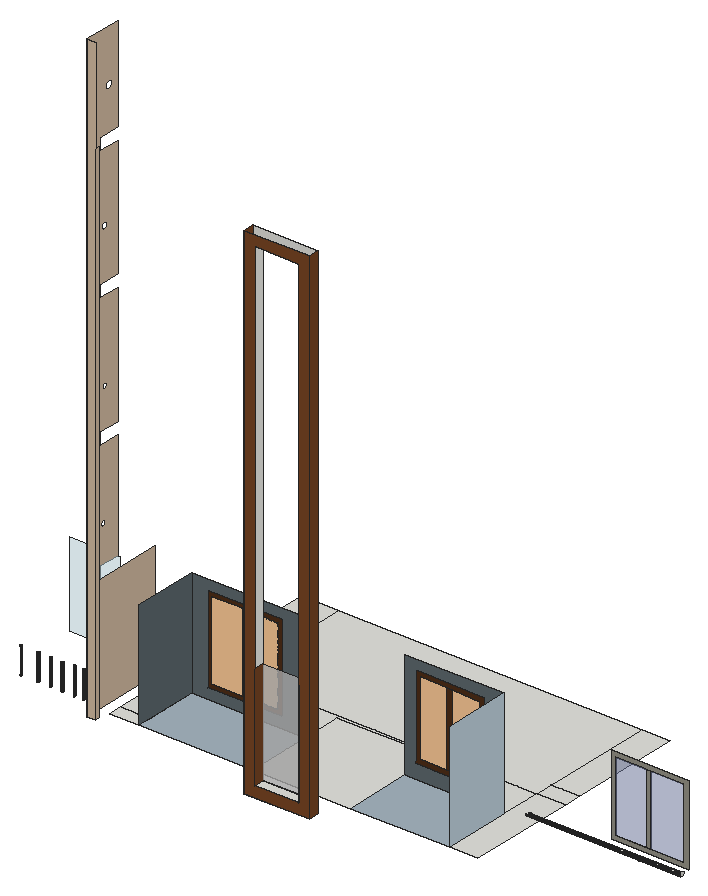
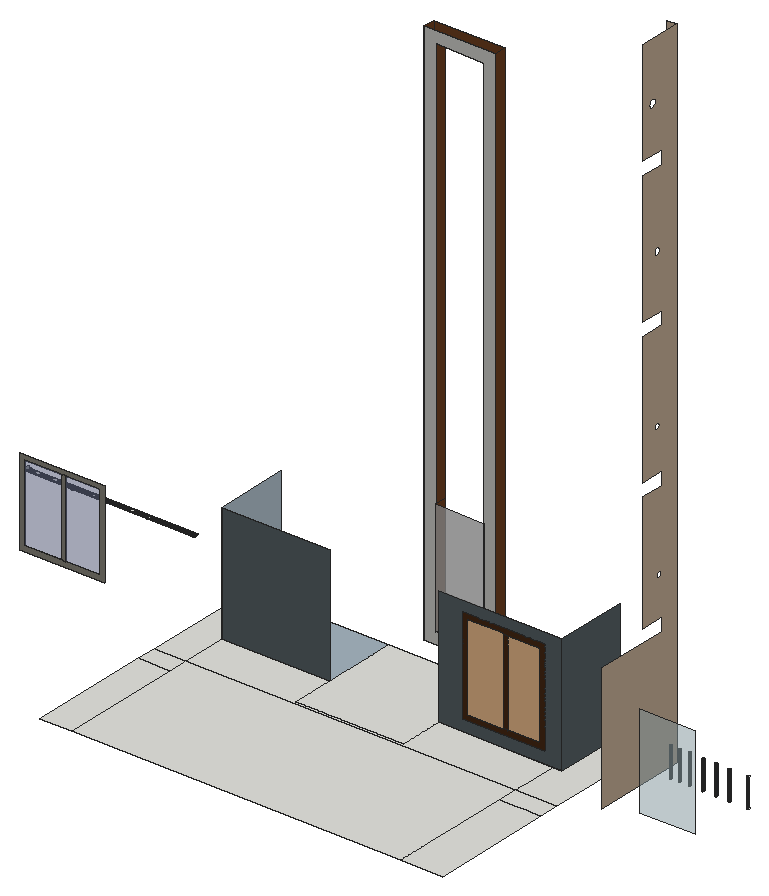
# SketchUp Ruby script. Lengths in inches.
U = 1.inch
M = Sketchup.active_model
def pt(a) = Geom::Point3d.new(a.map { |v| v * U })
def face(e, loops, mat)
  f = e.add_face(loops[0].map { |a| pt(a) })
  loops[1..].each { |l| e.add_face(l.map { |a| pt(a) }).erase! }
  f.material = f.back_material = mat if mat
  f
end
# faces: each face lists its corners as indices into pts; further lists are holes
def faces(e, pts, list, mat = nil) = list.each { |f| face(e, (f[0].is_a?(Array) ? f : [f]).map { |l| l.map { |i| pts[i] } }, mat) }
# xy, xz, yz: faces in a plane at the given z, y or x. An outline is a flat list of corners, or four numbers for a rectangle; further outlines are holes
def ring(l) = l.size == 4 ? [[l[0], l[1]], [l[2], l[1]], [l[2], l[3]], [l[0], l[3]]] : l.each_slice(2).to_a
def flat(e, list, mat, &to3) = list.each { |f| face(e, (f[0].is_a?(Array) ? f : [f]).map { |l| ring(l).map { |u, v| to3.(u, v) } }, mat) }
def xy(e, z, list, mat = nil) = flat(e, list, mat) { |x, y| [x, y, z] }
def xz(e, y, list, mat = nil) = flat(e, list, mat) { |x, z| [x, y, z] }
def yz(e, x, list, mat = nil) = flat(e, list, mat) { |y, z| [x, y, z] }
def lines(e, pts, list) = list.each { |a, b| e.add_line(pt(pts[a]), pt(pts[b])) }
# prism: a flat outline (further loops are holes) pulled along v
def prism(e, loops, v, mat = nil)
  f = face(e, loops, mat); d = Geom::Vector3d.new(v.map { |x| x * U })
  f.pushpull(f.normal.samedirection?(d) ? d.length : -d.length)
end
def box(e, o, s, mat = nil) = prism(e, [[o, [o[0] + s[0], o[1], o[2]], [o[0] + s[0], o[1] + s[1], o[2]], [o[0], o[1] + s[1], o[2]]]], [0, 0, s[2]], mat)
def at(x, y, z, deg = 0) = Geom::Transformation.translation(pt([x, y, z])) * Geom::Transformation.rotation(ORIGIN, Z_AXIS, deg.degrees)
def axes(o, x, y, z) = Geom::Transformation.new([*x, 0, *y, 0, *z, 0, *pt(o).to_a, 1])
def part(name) = M.definitions.add(name)
# library, detail: a bought-in or finely detailed component or shape, given as its bounding box
def library(name, o, s) = part(name).tap { |d| box(d.entities, o, s) }
def detail(e, o, s) = box(e.add_group.entities, o, s)
def put(e, d, t, mat = nil) = e.add_instance(d, t).tap { |i| i.material = mat if mat }
def group(e, t, mat = nil) = e.add_group.tap { |g| g.transformation = t; g.material = mat if mat }.entities
root = M.entities
M.materials.add("[Color C02]").color = [255, 204, 153]
M.materials.add("[Formica Graystone]").color = [149, 146, 135]
M.materials.add("[Formica Laminate Dark]").color = [50, 53, 60]
M.materials.add("[Formica Laminate Light]").color = [213, 189, 164]
M.materials.add("[Formica Speckled Grey]").color = [94, 105, 111]
M.materials.add("[Terrazzo Light Blue]1").color = [165, 180, 191]
M.materials.add("[Terrazzo Light Blue]2").color = [196, 214, 227]
M.materials.add("[Translucent Glass Safety]").color = [204, 235, 244]
M.materials["[Translucent Glass Safety]"].alpha = 0.5
M.materials.add("[Translucent Glass Sky Reflection]").color = [126, 138, 183]
M.materials["[Translucent Glass Sky Reflection]"].alpha = 0.52
M.materials.add("[Translucent Resin Crush Gray]").color = [201, 201, 201]
M.materials["[Translucent Resin Crush Gray]"].alpha = 0.8
M.materials.add("[Wood Veneer 01]").color = [79, 46, 24]
M.materials.add("[Wood Veneer 01]2").color = [120, 70, 37]
xy(root,133.5625,[[108.2,124.59,107.95,124.62,107.73,124.71,107.53,124.86,107.38,125.06,107.29,125.28,107.26,125.52,107.29,125.77,107.38,125.99,107.53,126.1875,107.73,126.34,107.95,126.43,108.2,126.46,108.4375,126.43,108.67,126.34,108.86,126.1875,109.01,125.99,109.1,125.77,109.13,125.52,109.1,125.28,109.01,125.06,108.86,124.86,108.67,124.71,108.4375,124.62],[125.32,124.59,125.08,124.62,124.85,124.71,124.66,124.86,124.51,125.06,124.42,125.28,124.38,125.52,124.42,125.77,124.51,125.99,124.66,126.1875,124.85,126.34,125.08,126.43,125.32,126.46,125.5625,126.43,125.79,126.34,125.98,126.1875,126.13,125.99,126.23,125.77,126.26,125.52,126.23,125.28,126.13,125.06,125.98,124.86,125.79,124.71,125.5625,124.62],[137.76,124.59,137.52,124.62,137.29,124.71,137.1,124.86,136.95,125.06,136.85,125.28,136.82,125.52,136.85,125.77,136.95,125.99,137.1,126.1875,137.29,126.34,137.52,126.43,137.76,126.46,138,126.43,138.23,126.34,138.42,126.1875,138.57,125.99,138.66,125.77,138.7,125.52,138.66,125.28,138.57,125.06,138.42,124.86,138.23,124.71,138,124.62],[149.57,124.59,149.33,124.62,149.1,124.71,148.91,124.86,148.76,125.06,148.67,125.28,148.63,125.52,148.67,125.77,148.76,125.99,148.91,126.1875,149.1,126.34,149.33,126.43,149.57,126.46,149.8125,126.43,150.04,126.34,150.23,126.1875,150.38,125.99,150.48,125.77,150.51,125.52,150.48,125.28,150.38,125.06,150.23,124.86,150.04,124.71,149.8125,124.62],[161.7,124.59,161.45,124.62,161.23,124.71,161.03,124.86,160.88,125.06,160.79,125.28,160.76,125.52,160.79,125.77,160.88,125.99,161.03,126.1875,161.23,126.34,161.45,126.43,161.7,126.46,161.9375,126.43,162.17,126.34,162.36,126.1875,162.51,125.99,162.6,125.77,162.63,125.52,162.6,125.28,162.51,125.06,162.36,124.86,162.17,124.71,161.9375,124.62],
  [170.82,124.59,170.58,124.62,170.35,124.71,170.16,124.86,170.01,125.06,169.92,125.28,169.88,125.52,169.92,125.77,170.01,125.99,170.16,126.1875,170.35,126.34,170.58,126.43,170.82,126.46,171.0625,126.43,171.29,126.34,171.48,126.1875,171.63,125.99,171.73,125.77,171.76,125.52,171.73,125.28,171.63,125.06,171.48,124.86,171.29,124.71,171.0625,124.62],[179.2,124.59,178.95,124.62,178.73,124.71,178.53,124.86,178.38,125.06,178.29,125.28,178.26,125.52,178.29,125.77,178.38,125.99,178.53,126.1875,178.73,126.34,178.95,126.43,179.2,126.46,179.4375,126.43,179.67,126.34,179.86,126.1875,180.01,125.99,180.1,125.77,180.13,125.52,180.1,125.28,180.01,125.06,179.86,124.86,179.67,124.71,179.4375,124.62]])
xy(root,140.5,[[369.87,77.26,435.37,88.2]])
xy(root,141,[[209,110.07,238.58,123.98],[351.88,110.07,450.54,216.34],[549.2,110.07,577.87,219.13],[209,123.98,238.58,123.98,238.58,175.78,246.77,175.78,246.77,219.13,209,219.13],[246.77,175.78,351.88,175.78,351.88,216.34,450.54,216.34,450.54,177.84,549.2,177.84,549.2,219.13,246.77,219.13],
  [209,219.13,246.77,237.1],[246.77,219.13,549.2,350.21],[549.2,219.13,577.87,237.1],[209,237.1,246.77,350.21],[549.2,237.1,577.87,350.21]])
xy(root,141,[[238.58,110.07,351.88,175.78],[450.54,110.07,549.2,177.84]],"[Terrazzo Light Blue]1")
xy(root,150.93,[[380.3,77.26,424.94,88.2]])
xy(root,159.6875,[[149.57,124.59,149.8125,124.62,150.04,124.71,150.23,124.86,150.38,125.06,150.48,125.28,150.51,125.52,150.48,125.77,150.38,125.99,150.23,126.1875,150.04,126.34,149.8125,126.43,149.57,126.46,149.33,126.43,149.1,126.34,148.91,126.1875,148.76,125.99,148.67,125.77,148.63,125.52,148.67,125.28,148.76,125.06,148.91,124.86,149.1,124.71,149.33,124.62]])
xy(root,159.875,[[125.32,124.59,125.5625,124.62,125.79,124.71,125.98,124.86,126.13,125.06,126.23,125.28,126.26,125.52,126.23,125.77,126.13,125.99,125.98,126.1875,125.79,126.34,125.5625,126.43,125.32,126.46,125.08,126.43,124.85,126.34,124.66,126.1875,124.51,125.99,124.42,125.77,124.38,125.52,124.42,125.28,124.51,125.06,124.66,124.86,124.85,124.71,125.08,124.62],[137.76,124.59,138,124.62,138.23,124.71,138.42,124.86,138.57,125.06,138.66,125.28,138.7,125.52,138.66,125.77,138.57,125.99,138.42,126.1875,138.23,126.34,138,126.43,137.76,126.46,137.52,126.43,137.29,126.34,137.1,126.1875,136.95,125.99,136.85,125.77,136.82,125.52,136.85,125.28,136.95,125.06,137.1,124.86,137.29,124.71,137.52,124.62]])
xy(root,160.125,[[108.2,124.59,108.4375,124.62,108.67,124.71,108.86,124.86,109.01,125.06,109.1,125.28,109.13,125.52,109.1,125.77,109.01,125.99,108.86,126.1875,108.67,126.34,108.4375,126.43,108.2,126.46,107.95,126.43,107.73,126.34,107.53,126.1875,107.38,125.99,107.29,125.77,107.26,125.52,107.29,125.28,107.38,125.06,107.53,124.86,107.73,124.71,107.95,124.62]])
xy(root,160.19,[[170.82,124.59,170.96,124.61,170.68,124.61],[170.68,124.61,170.96,124.61,171.0625,124.62,171.29,124.71,171.48,124.86,171.63,125.06,171.73,125.28,171.76,125.52,171.73,125.77,171.63,125.99,171.48,126.1875,171.29,126.34,171.0625,126.43,170.82,126.46,170.58,126.43,170.35,126.34,170.16,126.1875,170.01,125.99,169.92,125.77,169.88,125.52,169.92,125.28,170.01,125.06,170.16,124.86,170.35,124.71,170.58,124.62]])
xy(root,160.25,[[179.2,124.59,179.4375,124.62,179.67,124.71,179.86,124.86,180.01,125.06,180.1,125.28,180.13,125.52,180.1,125.77,180.01,125.99,179.86,126.1875,179.67,126.34,179.4375,126.43,179.2,126.46,178.95,126.43,178.73,126.34,178.53,126.1875,178.38,125.99,178.29,125.77,178.26,125.52,178.29,125.28,178.38,125.06,178.53,124.86,178.73,124.71,178.95,124.62]])
xy(root,160.5,[[161.7,124.59,161.9375,124.62,162.17,124.71,162.36,124.86,162.51,125.06,162.6,125.28,162.63,125.52,162.6,125.77,162.51,125.99,162.36,126.1875,162.17,126.34,161.9375,126.43,161.7,126.46,161.45,126.43,161.23,126.34,161.03,126.1875,160.88,125.99,160.79,125.77,160.76,125.52,160.79,125.28,160.88,125.06,161.03,124.86,161.23,124.71,161.45,124.62]])
xy(root,182,[[723.39,128.83,723.78,128.89,724.14,129.04,724.45,129.27,724.6875,129.58,724.84,129.95,724.89,130.33,724.84,130.72,724.6875,131.08,724.45,131.4,724.14,131.63,723.78,131.78,723.39,131.83,723,131.78,722.64,131.63,722.33,131.4,722.09,131.08,721.9375,130.72,721.89,130.33,721.9375,129.95,722.09,129.58,722.33,129.27,722.64,129.04,723,128.89]])
xy(root,182.75,[[654.01,128.83,654.4,128.89,654.76,129.04,655.07,129.27,655.3125,129.58,655.46,129.95,655.51,130.33,655.46,130.72,655.3125,131.08,655.07,131.4,654.76,131.63,654.4,131.78,654.01,131.83,653.625,131.78,653.26,131.63,652.95,131.4,652.71,131.08,652.5625,130.72,652.51,130.33,652.5625,129.95,652.71,129.58,652.95,129.27,653.26,129.04,653.625,128.89]])
xy(root,182.9375,[[669.45,128.83,669.84,128.89,670.2,129.04,670.51,129.27,670.75,129.58,670.9,129.95,670.95,130.33,670.9,130.72,670.75,131.08,670.51,131.4,670.2,131.63,669.84,131.78,669.45,131.83,669.0625,131.78,668.7,131.63,668.39,131.4,668.15,131.08,668,130.72,667.95,130.33,668,129.95,668.15,129.58,668.39,129.27,668.7,129.04,669.0625,128.89]])
xy(root,183.1875,[[704.89,128.83,705.28,128.89,705.64,129.04,705.95,129.27,706.1875,129.58,706.34,129.95,706.39,130.33,706.34,130.72,706.1875,131.08,705.95,131.4,705.64,131.63,705.28,131.78,704.89,131.83,704.5,131.78,704.14,131.63,703.83,131.4,703.59,131.08,703.4375,130.72,703.39,130.33,703.4375,129.95,703.59,129.58,703.83,129.27,704.14,129.04,704.5,128.89]])
xy(root,183.5625,[[740.01,128.83,740.4,128.89,740.76,129.04,741.07,129.27,741.3125,129.58,741.46,129.95,741.51,130.33,741.46,130.72,741.3125,131.08,741.07,131.4,740.76,131.63,740.4,131.78,740.01,131.83,739.625,131.78,739.26,131.63,738.95,131.4,738.71,131.08,738.5625,130.72,738.51,130.33,738.5625,129.95,738.71,129.58,738.95,129.27,739.26,129.04,739.625,128.89],[756.14,128.83,756.53,128.89,756.89,129.04,757.2,129.27,757.4375,129.58,757.59,129.95,757.64,130.33,757.59,130.72,757.4375,131.08,757.2,131.4,756.89,131.63,756.53,131.78,756.14,131.83,755.75,131.78,755.39,131.63,755.08,131.4,754.84,131.08,754.6875,130.72,754.64,130.33,754.6875,129.95,754.84,129.58,755.08,129.27,755.39,129.04,755.75,128.89]])
xz(root,77.26,[[[369.87,140.5,435.37,645],[380.3,150.93,424.94,634.57]]],"[Wood Veneer 01]2")
xz(root,88.2,[[[369.87,140.5,435.37,645],[380.3,150.93,424.94,634.57]]])
xz(root,88.2,[[380.3,150.93,424.94,255.83]],"[Translucent Resin Crush Gray]")
xz(root,105.54,[[189.57,133.5625,198.57,740.5625]],"[Formica Laminate Light]")
xz(root,175.78,[[259.03,156.3,288.77,234.59],[293.54,156.3,324.94,234.59]],"[Color C02]")
xz(root,175.78,[[[238.58,141,351.88,249],[254.45,151.72,329.52,239.16]]],"[Formica Speckled Grey]")
xz(root,175.78,[[[254.45,151.72,329.52,239.16],[259.03,156.3,324.94,234.59]],[288.77,156.3,293.54,234.59]],"[Wood Veneer 01]")
xz(root,177.84,[[450.54,141,549.2,249]],"[Formica Speckled Grey]")
xz(root,182.57,[[[653.07,152.76,730.45,232.51],[657.67,157.36,725.85,227.92]],[688.06,157.36,692.49,227.92]],"[Formica Graystone]")
xz(root,182.57,[[657.67,157.36,688.06,227.92],[692.49,157.36,725.85,227.92]],"[Translucent Glass Sky Reflection]")
xz(root,191.15,[[104.16,141.71,155.34,227.3]],"[Translucent Glass Safety]")
yz(root,189.57,[[[105.54,133.5625,105.54,740.5625,144.21,740.5625,144.21,645,122.79,645,122.79,633,144.21,633,144.21,513,122.79,513,122.79,501,144.21,501,144.21,381,122.79,381,122.79,369,144.21,369,144.21,261,122.79,261,122.79,249,191.15,249,191.15,133.5625],[133.5,683.96,134.47,684.08,135.38,684.46,136.15,685.06,136.75,685.83,137.125,686.74,137.25,687.71,137.125,688.68,136.75,689.58,136.15,690.36,135.38,690.95,134.47,691.33,133.5,691.46,132.53,691.33,131.63,690.95,130.85,690.36,130.25,689.58,129.88,688.68,129.75,687.71,129.88,686.74,130.25,685.83,130.85,685.06,131.63,684.46,132.53,684.08],[128.15,560.5625,128.99,560.67,129.77,561,130.45,561.51,130.96,562.1875,131.29,562.97,131.4,563.8125,131.29,564.65,130.96,565.4375,130.45,566.11,129.77,566.625,128.99,566.95,128.15,567.0625,127.31,566.95,126.52,566.625,125.85,566.11,125.33,565.4375,125.01,564.65,124.9,563.8125,125.01,562.97,125.33,562.1875,125.85,561.51,126.52,561,127.31,560.67],[126.49,294.81,127.1875,294.9,127.84,295.17,128.39,295.59,128.82,296.15,129.09,296.8,129.18,297.49,129.09,298.1875,128.82,298.84,128.39,299.39,127.84,299.82,127.1875,300.09,126.49,300.18,125.8,300.09,125.15,299.82,124.59,299.39,124.17,298.84,123.9,298.1875,123.81,297.49,123.9,296.8,124.17,296.15,124.59,295.59,125.15,295.17,125.8,294.9],[128.15,417.26,128.84,417.35,129.49,417.625,130.05,418.05,130.48,418.61,130.74,419.26,130.84,419.95,130.74,420.65,130.48,421.29,130.05,421.85,129.49,422.28,128.84,422.55,128.15,422.64,127.45,422.55,126.8,422.28,126.25,421.85,125.82,421.29,125.55,420.65,125.46,419.95,125.55,419.26,125.82,418.61,126.25,418.05,126.8,417.625,127.45,417.35],[125.67,159.02,125.92,159.07,126.16,159.1875,126.35,159.36,126.49,159.58,126.57,159.83,126.59,160.09,126.53,160.35,126.41,160.58,126.24,160.77,126.02,160.92,125.77,161,125.51,161.01,125.26,160.96,125.02,160.84,124.83,160.66,124.6875,160.44,124.61,160.19,124.59,159.93,124.65,159.68,124.77,159.45,124.94,159.25,125.16,159.11,125.41,159.03]]],"[Formica Laminate Light]")
yz(root,198.57,[[105.54,133.5625,110.07,645]],"[Formica Laminate Light]")
yz(root,238.58,[[110.07,141,175.78,249]],"[Formica Speckled Grey]")
yz(root,369.87,[[77.26,140.5,88.2,645]],"[Wood Veneer 01]2")
yz(root,380.3,[[77.26,150.93,88.2,255.83]],"[Wood Veneer 01]2")
yz(root,424.94,[[77.26,150.93,88.2,255.83]],"[Wood Veneer 01]2")
yz(root,435.37,[[77.26,140.5,88.2,645]],"[Wood Veneer 01]2")
yz(root,549.2,[[110.07,141,177.84,249]],"[Terrazzo Light Blue]2")
yz(root,765.67,[[130.24,182.07,130.76,182.14,131.24,182.34,131.66,182.66,131.98,183.07,132.18,183.55,132.24,184.07,132.18,184.59,131.98,185.07,131.66,185.49,131.24,185.8,130.76,186,130.24,186.07,129.73,186,129.24,185.8,128.83,185.49,128.51,185.07,128.3125,184.59,128.24,184.07,128.3125,183.55,128.51,183.07,128.83,182.66,129.24,182.34,129.73,182.14]])
p = [[108.2,124.59,133.5625],[108.4375,124.62,133.5625],[108.4375,124.62,160.125],[108.2,124.59,160.125],[108.67,124.71,133.5625],[108.67,124.71,160.125],
  [124.85,124.71,133.5625],[125.08,124.62,133.5625],[125.08,124.62,159.875],[124.85,124.71,159.875],[125.32,124.59,133.5625],[125.32,124.59,159.875],
  [125.5625,124.62,133.5625],[125.5625,124.62,159.875],[125.79,124.71,133.5625],[125.79,124.71,159.875],[137.29,124.71,133.5625],[137.52,124.62,133.5625],
  [137.52,124.62,159.875],[137.29,124.71,159.875],[137.76,124.59,133.5625],[137.76,124.59,159.875],[138,124.62,133.5625],[138,124.62,159.875],
  [138.23,124.71,133.5625],[138.23,124.71,159.875],[149.1,124.71,133.5625],[149.33,124.62,133.5625],[149.33,124.62,159.6875],[149.1,124.71,159.6875],
  [149.57,124.59,133.5625],[149.57,124.59,159.6875],[149.8125,124.62,133.5625],[149.8125,124.62,159.6875],[150.04,124.71,133.5625],[150.04,124.71,159.6875],
  [161.23,124.71,133.5625],[161.45,124.62,133.5625],[161.45,124.62,160.5],[161.23,124.71,160.5],[161.7,124.59,133.5625],[161.7,124.59,160.5],
  [161.9375,124.62,133.5625],[161.9375,124.62,160.5],[162.17,124.71,133.5625],[162.17,124.71,160.5],[170.35,124.71,133.5625],[170.58,124.62,133.5625],
  [170.58,124.62,160.19],[170.35,124.71,160.19],[170.82,124.59,133.5625],[170.82,124.59,160.19],[170.68,124.61,160.19],[171.0625,124.62,133.5625],
  [171.0625,124.62,160.19],[170.96,124.61,160.19],[171.29,124.71,133.5625],[171.29,124.71,160.19],[178.73,124.71,133.5625],[178.95,124.62,133.5625],
  [178.95,124.62,160.25],[178.73,124.71,160.25],[179.2,124.59,133.5625],[179.2,124.59,160.25],[179.4375,124.62,133.5625],[179.4375,124.62,160.25],
  [179.67,124.71,133.5625],[179.67,124.71,160.25],[108.86,124.86,133.5625],[108.86,124.86,160.125],[124.66,124.86,133.5625],[124.66,124.86,159.875],
  [125.98,124.86,133.5625],[125.98,124.86,159.875],[137.1,124.86,133.5625],[137.1,124.86,159.875],[138.42,124.86,133.5625],[138.42,124.86,159.875],
  [148.91,124.86,133.5625],[148.91,124.86,159.6875],[150.23,124.86,133.5625],[150.23,124.86,159.6875],[161.03,124.86,133.5625],[161.03,124.86,160.5],
  [162.36,124.86,133.5625],[162.36,124.86,160.5],[170.16,124.86,133.5625],[170.16,124.86,160.19],[171.48,124.86,133.5625],[171.48,124.86,160.19],
  [178.53,124.86,133.5625],[178.53,124.86,160.25],[179.86,124.86,133.5625],[179.86,124.86,160.25],[109.01,125.06,133.5625],[109.01,125.06,160.125],
  [124.51,125.06,133.5625],[124.51,125.06,159.875],[126.13,125.06,133.5625],[126.13,125.06,159.875],[136.95,125.06,133.5625],[136.95,125.06,159.875],
  [138.57,125.06,133.5625],[138.57,125.06,159.875],[148.76,125.06,133.5625],[148.76,125.06,159.6875],[150.38,125.06,133.5625],[150.38,125.06,159.6875],
  [160.88,125.06,133.5625],[160.88,125.06,160.5],[162.51,125.06,133.5625],[162.51,125.06,160.5],[170.01,125.06,133.5625],[170.01,125.06,160.19],
  [171.63,125.06,133.5625],[171.63,125.06,160.19],[178.38,125.06,133.5625],[178.38,125.06,160.25],[180.01,125.06,133.5625],[180.01,125.06,160.25],
  [109.1,125.28,133.5625],[109.1,125.28,160.125],[124.42,125.28,133.5625],[124.42,125.28,159.875],[126.23,125.28,133.5625],[126.23,125.28,159.875],
  [136.85,125.28,133.5625],[136.85,125.28,159.875],[138.66,125.28,133.5625],[138.66,125.28,159.875],[148.67,125.28,133.5625],[148.67,125.28,159.6875],
  [150.48,125.28,133.5625],[150.48,125.28,159.6875],[160.79,125.28,133.5625],[160.79,125.28,160.5],[162.6,125.28,133.5625],[162.6,125.28,160.5],
  [169.92,125.28,133.5625],[169.92,125.28,160.19],[171.73,125.28,133.5625],[171.73,125.28,160.19],[178.29,125.28,133.5625],[178.29,125.28,160.25],
  [180.1,125.28,133.5625],[180.1,125.28,160.25],[109.13,125.52,133.5625],[109.13,125.52,160.125],[124.38,125.52,133.5625],[124.38,125.52,159.875],
  [126.26,125.52,133.5625],[126.26,125.52,159.875],[136.82,125.52,133.5625],[136.82,125.52,159.875],[138.7,125.52,133.5625],[138.7,125.52,159.875],
  [148.63,125.52,133.5625],[148.63,125.52,159.6875],[150.51,125.52,133.5625],[150.51,125.52,159.6875],[160.76,125.52,133.5625],[160.76,125.52,160.5],
  [162.63,125.52,133.5625],[162.63,125.52,160.5],[169.88,125.52,133.5625],[169.88,125.52,160.19],[171.76,125.52,133.5625],[171.76,125.52,160.19],
  [178.26,125.52,133.5625],[178.26,125.52,160.25],[180.13,125.52,133.5625],[180.13,125.52,160.25],[109.1,125.77,133.5625],[109.1,125.77,160.125],
  [124.42,125.77,133.5625],[124.42,125.77,159.875],[126.23,125.77,133.5625],[126.23,125.77,159.875],[136.85,125.77,133.5625],[136.85,125.77,159.875],
  [138.66,125.77,133.5625],[138.66,125.77,159.875],[148.67,125.77,133.5625],[148.67,125.77,159.6875],[150.48,125.77,133.5625],[150.48,125.77,159.6875],
  [160.79,125.77,133.5625],[160.79,125.77,160.5],[162.6,125.77,133.5625],[162.6,125.77,160.5],[169.92,125.77,133.5625],[169.92,125.77,160.19],
  [171.73,125.77,133.5625],[171.73,125.77,160.19],[178.29,125.77,133.5625],[178.29,125.77,160.25],[180.1,125.77,133.5625],[180.1,125.77,160.25],
  [109.01,125.99,133.5625],[109.01,125.99,160.125],[124.51,125.99,133.5625],[124.51,125.99,159.875],[126.13,125.99,133.5625],[126.13,125.99,159.875],
  [136.95,125.99,133.5625],[136.95,125.99,159.875],[138.57,125.99,133.5625],[138.57,125.99,159.875],[148.76,125.99,133.5625],[148.76,125.99,159.6875],
  [150.38,125.99,133.5625],[150.38,125.99,159.6875],[160.88,125.99,133.5625],[160.88,125.99,160.5],[162.51,125.99,133.5625],[162.51,125.99,160.5],
  [170.01,125.99,133.5625],[170.01,125.99,160.19],[171.63,125.99,133.5625],[171.63,125.99,160.19],[178.38,125.99,133.5625],[178.38,125.99,160.25],
  [180.01,125.99,133.5625],[180.01,125.99,160.25],[108.86,126.1875,133.5625],[108.86,126.1875,160.125],[124.66,126.1875,133.5625],[124.66,126.1875,159.875],
  [125.98,126.1875,133.5625],[125.98,126.1875,159.875],[137.1,126.1875,133.5625],[137.1,126.1875,159.875],[138.42,126.1875,133.5625],[138.42,126.1875,159.875],
  [148.91,126.1875,133.5625],[148.91,126.1875,159.6875],[150.23,126.1875,133.5625],[150.23,126.1875,159.6875],[161.03,126.1875,133.5625],[161.03,126.1875,160.5],
  [162.36,126.1875,133.5625],[162.36,126.1875,160.5],[170.16,126.1875,133.5625],[170.16,126.1875,160.19],[171.48,126.1875,133.5625],[171.48,126.1875,160.19],
  [178.53,126.1875,133.5625],[178.53,126.1875,160.25],[179.86,126.1875,133.5625],[179.86,126.1875,160.25],[108.67,126.34,133.5625],[108.67,126.34,160.125],
  [124.85,126.34,133.5625],[124.85,126.34,159.875],[125.79,126.34,133.5625],[125.79,126.34,159.875],[137.29,126.34,133.5625],[137.29,126.34,159.875],
  [138.23,126.34,133.5625],[138.23,126.34,159.875],[149.1,126.34,133.5625],[149.1,126.34,159.6875],[150.04,126.34,133.5625],[150.04,126.34,159.6875],
  [161.23,126.34,133.5625],[161.23,126.34,160.5],[162.17,126.34,133.5625],[162.17,126.34,160.5],[170.35,126.34,133.5625],[170.35,126.34,160.19],
  [171.29,126.34,133.5625],[171.29,126.34,160.19],[178.73,126.34,133.5625],[178.73,126.34,160.25],[179.67,126.34,133.5625],[179.67,126.34,160.25],
  [108.4375,126.43,133.5625],[108.4375,126.43,160.125],[125.08,126.43,133.5625],[125.08,126.43,159.875],[125.5625,126.43,133.5625],[125.5625,126.43,159.875],
  [137.52,126.43,133.5625],[137.52,126.43,159.875],[138,126.43,133.5625],[138,126.43,159.875],[149.33,126.43,133.5625],[149.33,126.43,159.6875],
  [149.8125,126.43,133.5625],[149.8125,126.43,159.6875],[161.45,126.43,133.5625],[161.45,126.43,160.5],[161.9375,126.43,133.5625],[161.9375,126.43,160.5],
  [170.58,126.43,133.5625],[170.58,126.43,160.19],[171.0625,126.43,133.5625],[171.0625,126.43,160.19],[178.95,126.43,133.5625],[178.95,126.43,160.25],
  [179.4375,126.43,133.5625],[179.4375,126.43,160.25],[108.2,126.46,133.5625],[107.95,126.43,133.5625],[107.95,126.43,160.125],[108.2,126.46,160.125],
  [125.32,126.46,133.5625],[125.32,126.46,159.875],[137.76,126.46,133.5625],[137.76,126.46,159.875],[149.57,126.46,133.5625],[149.57,126.46,159.6875],
  [161.7,126.46,133.5625],[161.7,126.46,160.5],[170.82,126.46,133.5625],[170.82,126.46,160.19],[179.2,126.46,133.5625],[179.2,126.46,160.25],
  [461.54,177.84,239.2],[461.54,177.84,156.3],[531.08,175.78,156.3],[531.08,175.78,239.2],[526.21,175.92,234.33],[526.21,175.92,161.16],
  [497.94,176.76,161.16],[493.09,176.9,161.16],[466.4,177.69,161.16],[466.4,177.69,234.33],[493.09,176.9,234.33],[497.94,176.76,234.33],
  [765.67,129.73,182.14],[765.67,129.24,182.34],[611.125,129.24,182.34],[611.125,129.73,182.14],[765.67,130.24,182.07],[611.125,130.24,182.07],
  [765.67,130.76,182.14],[611.125,130.76,182.14],[765.67,131.24,182.34],[611.125,131.24,182.34],[765.67,128.83,182.66],[611.125,128.83,182.66],
  [765.67,131.66,182.66],[611.125,131.66,182.66],[765.67,128.51,183.07],[611.125,128.51,183.07],[765.67,131.98,183.07],[611.125,131.98,183.07],
  [765.67,128.3125,183.55],[611.125,128.3125,183.55],[765.67,132.18,183.55],[611.125,132.18,183.55],[765.67,128.24,184.07],[611.125,128.24,184.07],
  [765.67,132.24,184.07],[611.125,132.24,184.07]]
faces(root,p,[[0,1,2,3],[1,4,5,2],[6,7,8,9],[7,10,11,8],[10,12,13,11],[12,14,15,13],[16,17,18,19],[17,20,21,18],
  [20,22,23,21],[22,24,25,23],[26,27,28,29],[27,30,31,28],[30,32,33,31],[32,34,35,33],[36,37,38,39],[37,40,41,38],
  [40,42,43,41],[42,44,45,43],[46,47,48,49],[47,50,51,52,48],[50,53,54,55,51],[53,56,57,54],[58,59,60,61],[59,62,63,60],
  [62,64,65,63],[64,66,67,65],[4,68,69,5],[70,6,9,71],[14,72,73,15],[74,16,19,75],[24,76,77,25],[78,26,29,79],
  [34,80,81,35],[82,36,39,83],[44,84,85,45],[86,46,49,87],[56,88,89,57],[90,58,61,91],[66,92,93,67],[68,94,95,69],
  [96,70,71,97],[72,98,99,73],[100,74,75,101],[76,102,103,77],[104,78,79,105],[80,106,107,81],[108,82,83,109],[84,110,111,85],
  [112,86,87,113],[88,114,115,89],[116,90,91,117],[92,118,119,93],[94,120,121,95],[122,96,97,123],[98,124,125,99],[126,100,101,127],
  [102,128,129,103],[130,104,105,131],[106,132,133,107],[134,108,109,135],[110,136,137,111],[138,112,113,139],[114,140,141,115],[142,116,117,143],
  [118,144,145,119],[120,146,147,121],[148,122,123,149],[124,150,151,125],[152,126,127,153],[128,154,155,129],[156,130,131,157],[132,158,159,133],
  [160,134,135,161],[136,162,163,137],[164,138,139,165],[140,166,167,141],[168,142,143,169],[144,170,171,145],[146,172,173,147],[174,148,149,175],
  [150,176,177,151],[178,152,153,179],[154,180,181,155],[182,156,157,183],[158,184,185,159],[186,160,161,187],[162,188,189,163],[190,164,165,191],
  [166,192,193,167],[194,168,169,195],[170,196,197,171],[172,198,199,173],[200,174,175,201],[176,202,203,177],[204,178,179,205],[180,206,207,181],
  [208,182,183,209],[184,210,211,185],[212,186,187,213],[188,214,215,189],[216,190,191,217],[192,218,219,193],[220,194,195,221],[196,222,223,197],
  [198,224,225,199],[226,200,201,227],[202,228,229,203],[230,204,205,231],[206,232,233,207],[234,208,209,235],[210,236,237,211],[238,212,213,239],
  [214,240,241,215],[242,216,217,243],[218,244,245,219],[246,220,221,247],[222,248,249,223],[224,250,251,225],[252,226,227,253],[228,254,255,229],
  [256,230,231,257],[232,258,259,233],[260,234,235,261],[236,262,263,237],[264,238,239,265],[240,266,267,241],[268,242,243,269],[244,270,271,245],
  [272,246,247,273],[248,274,275,249],[250,276,277,251],[278,252,253,279],[254,280,281,255],[282,256,257,283],[258,284,285,259],[286,260,261,287],
  [262,288,289,263],[290,264,265,291],[266,292,293,267],[294,268,269,295],[270,296,297,271],[298,272,273,299],[274,300,301,275],[302,303,304,305],
  [276,302,305,277],[306,278,279,307],[280,306,307,281],[308,282,283,309],[284,308,309,285],[310,286,287,311],[288,310,311,289],[312,290,291,313],
  [292,312,313,293],[314,294,295,315],[296,314,315,297],[316,298,299,317],[300,316,317,301],[330,331,332,333],[334,330,333,335],[336,334,335,337],
  [338,336,337,339],[331,340,341,332],[342,338,339,343],[340,344,345,341],[346,342,343,347],[344,348,349,345],[350,346,347,351],[348,352,353,349],
  [354,350,351,355]],"[Formica Laminate Dark]")
faces(root,p,[[[318,319,320,321],[322,323,324,325,326,327,328,329]],[325,324,329,328]],"[Wood Veneer 01]")
faces(root,p,[[322,329,324,323],[326,325,328,327]],"[Color C02]")
